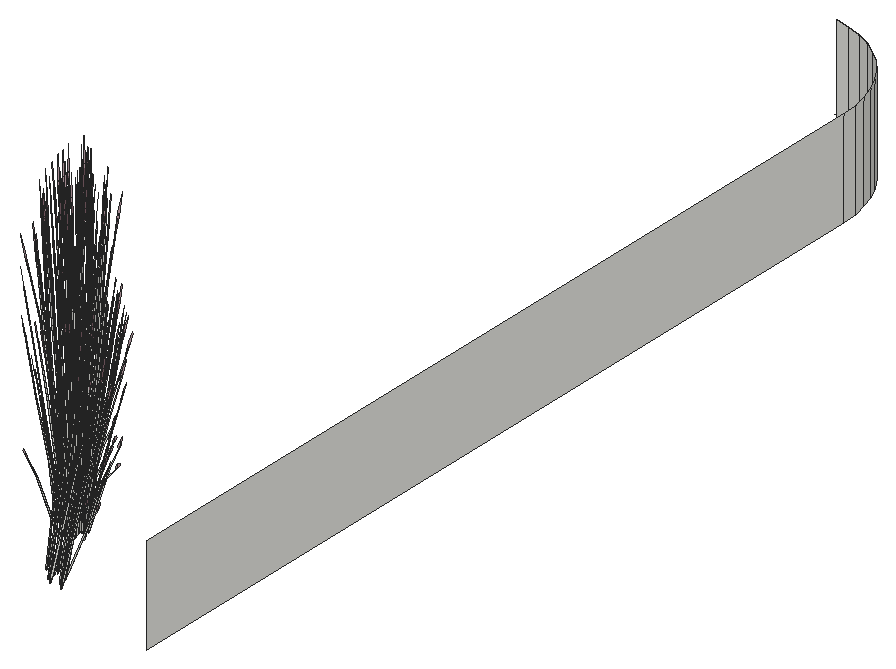
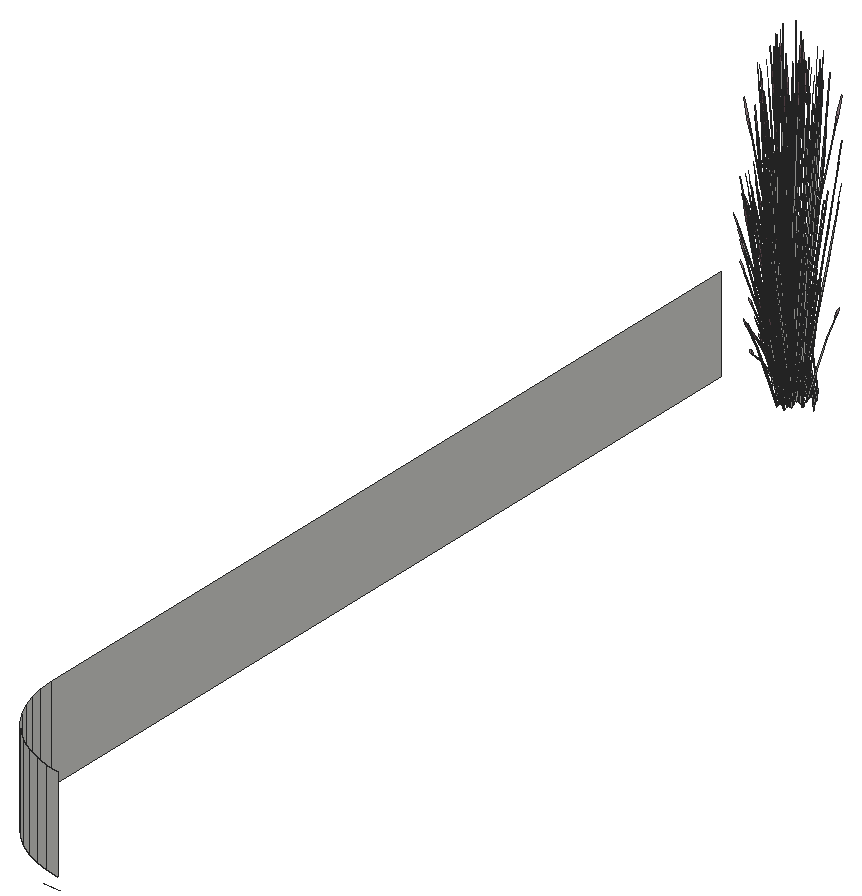
# SketchUp Ruby script. Lengths in inches.
U = 1.inch
M = Sketchup.active_model
def pt(a) = Geom::Point3d.new(a.map { |v| v * U })
def face(e, loops, mat)
  f = e.add_face(loops[0].map { |a| pt(a) })
  loops[1..].each { |l| e.add_face(l.map { |a| pt(a) }).erase! }
  f.material = f.back_material = mat if mat
  f
end
# faces: each face lists its corners as indices into pts; further lists are holes
def faces(e, pts, list, mat = nil) = list.each { |f| face(e, (f[0].is_a?(Array) ? f : [f]).map { |l| l.map { |i| pts[i] } }, mat) }
# xy, xz, yz: faces in a plane at the given z, y or x. An outline is a flat list of corners, or four numbers for a rectangle; further outlines are holes
def ring(l) = l.size == 4 ? [[l[0], l[1]], [l[2], l[1]], [l[2], l[3]], [l[0], l[3]]] : l.each_slice(2).to_a
def flat(e, list, mat, &to3) = list.each { |f| face(e, (f[0].is_a?(Array) ? f : [f]).map { |l| ring(l).map { |u, v| to3.(u, v) } }, mat) }
def xy(e, z, list, mat = nil) = flat(e, list, mat) { |x, y| [x, y, z] }
def xz(e, y, list, mat = nil) = flat(e, list, mat) { |x, z| [x, y, z] }
def yz(e, x, list, mat = nil) = flat(e, list, mat) { |y, z| [x, y, z] }
def lines(e, pts, list) = list.each { |a, b| e.add_line(pt(pts[a]), pt(pts[b])) }
# prism: a flat outline (further loops are holes) pulled along v
def prism(e, loops, v, mat = nil)
  f = face(e, loops, mat); d = Geom::Vector3d.new(v.map { |x| x * U })
  f.pushpull(f.normal.samedirection?(d) ? d.length : -d.length)
end
def box(e, o, s, mat = nil) = prism(e, [[o, [o[0] + s[0], o[1], o[2]], [o[0] + s[0], o[1] + s[1], o[2]], [o[0], o[1] + s[1], o[2]]]], [0, 0, s[2]], mat)
def at(x, y, z, deg = 0) = Geom::Transformation.translation(pt([x, y, z])) * Geom::Transformation.rotation(ORIGIN, Z_AXIS, deg.degrees)
def axes(o, x, y, z) = Geom::Transformation.new([*x, 0, *y, 0, *z, 0, *pt(o).to_a, 1])
def part(name) = M.definitions.add(name)
# library, detail: a bought-in or finely detailed component or shape, given as its bounding box
def library(name, o, s) = part(name).tap { |d| box(d.entities, o, s) }
def detail(e, o, s) = box(e.add_group.entities, o, s)
def put(e, d, t, mat = nil) = e.add_instance(d, t).tap { |i| i.material = mat if mat }
def group(e, t, mat = nil) = e.add_group.tap { |g| g.transformation = t; g.material = mat if mat }.entities
root = M.entities
M.materials.add("LightPink_Translucent").color = [144, 107, 117]
M.materials["LightPink_Translucent"].alpha = 0.75
c1 = part("blade")
p = [[2.15,0.21,22],[0,0.17,0],[0.09,0.45,0],[2.18,0.31,22],[2.29,0.31,22],[0.38,0.45,0],
  [2.48,0.24,33],[2.49,0.24,33],[2.48,0.22,33]]
faces(c1.entities,p,[[0,1,2,3],[4,5,2,3],[6,3,4,7],[8,0,3,6]])
c2 = part("seeds")
p = [[0.3,-0.1,1.38],[-0.01,-0.03,1.59],[-0.01,-0.03,0.03],[0.14,-0.07,-0.07],[0.29,-0.03,3],[0.15,0.01,3.11]]
faces(c2.entities,p,[[0,1,2,3],[1,0,4,5]],"LightPink_Translucent")
c3 = part("blade with seeds")
put(c3.entities,c1,at(0,0,0))
put(c3.entities,c2,axes([2.4,0.25,30.99],[1.5799,-0.05474,1.17369],[-0.12525,1.92788,0.29478],[-0.07173,-0.02425,1.56792]))
yz(root,375.57,[[661.9,618,822.84,636]])
p = [[375.39,825.68,618],[375.57,822.84,618],[375.57,822.84,636],[375.39,825.68,636],[374.85,828.375,618],[374.85,828.375,636],
  [373.97,830.97,618],[373.97,830.97,636],[372.76,833.4375,618],[372.76,833.4375,636],[371.23,835.72,618],[371.23,835.72,636],
  [369.42,837.79,618],[369.42,837.79,636],[367.36,839.6,618],[367.36,839.6,636],[365.07,841.12,618],[365.07,841.12,636],
  [362.61,842.34,618],[362.61,842.34,636],[360.01,843.22,618],[360.01,843.22,636],[357.59,843.7,618],[357.59,843.7,636],
  [357.71,846.74,618],[354.57,846.94,618],[357.88,846.7,618]]
faces(root,p,[[0,1,2,3],[4,0,3,5],[6,4,5,7],[8,6,7,9],[10,8,9,11],[12,10,11,13],[14,12,13,15],[16,14,15,17],
  [18,16,17,19],[20,18,19,21],[22,20,21,23]])
lines(root,p,[[24,25],[26,24]])
put(root,c3,axes([356.22,664.375,622.68],[0.34695,0.11691,-0.51099],[-0.11892,0.40083,-0.3958],[0.03181,0.16138,0.97773]))
put(root,c3,axes([357.33,664.56,620.82],[0.32063,-0.08258,0.06507],[0.07371,0.33271,-0.86304],[-0.02033,0.16842,0.7736]))
put(root,c3,axes([356.42,663.55,621.875],[-0.08068,-0.14973,1.71376],[0.3728,-0.12606,0.13857],[0.08426,0.23506,0.73262]))
put(root,c3,axes([358.35,664.39,622.68],[0.34695,0.11691,-0.51099],[-0.11892,0.40083,-0.3958],[0.03181,0.16138,0.97773]))
put(root,c3,axes([358.55,663.5625,621.875],[-0.08068,-0.14973,1.71376],[0.3728,-0.12606,0.13857],[0.08426,0.23506,0.73262]))
put(root,c3,axes([353.5,669.76,628.32],[0.16041,-0.29625,0.0643],[0.22843,0.17248,0.50621],[-0.07385,-0.09498,0.77189]))
put(root,c3,axes([352.875,669.72,625.08],[-0.03419,0.06144,1.76342],[-0.3455,0.13246,-0.26939],[-0.08346,-0.12049,0.30037]))
put(root,c3,axes([356.0625,664.62,622.53],[-0.1064,0.35863,-0.35414],[-0.31043,-0.1046,0.4572],[0.02846,0.14439,0.87481]))
put(root,c3,axes([358.19,664.63,622.53],[-0.1064,0.35863,-0.35414],[-0.31043,-0.1046,0.4572],[0.02846,0.14439,0.87481]))
put(root,c3,axes([353.44,671.41,625.6875],[-0.14494,-0.47823,-0.69835],[0.41752,-0.17223,-0.18329],[-0.01602,-0.16194,1.54149]))
put(root,c3,axes([355.38,669.95,625.08],[-0.05283,-0.03674,1.76342],[-0.13569,-0.41045,-0.26939],[0.09154,-0.11138,0.30037]))
put(root,c3,axes([355.39,663.93,623.34],[-0.00918,0.43138,-0.7886],[-0.38672,-0.02897,0.09517],[-0.04081,0.18275,1.11556]))
put(root,c3,axes([357.52,663.94,623.34],[-0.00918,0.43138,-0.7886],[-0.38672,-0.02897,0.09517],[-0.04081,0.18275,1.11556]))
put(root,c3,axes([354.38,665.06,622.71],[0.04004,-0.02816,1.77383],[0.33095,0.18728,-0.16761],[-0.00778,0.15594,0.31391]))
put(root,c3,axes([356.51,665.07,622.71],[0.04004,-0.02816,1.77383],[0.33095,0.18728,-0.16761],[-0.00778,0.15594,0.31391]))
put(root,c3,axes([354.29,670.04,628.64],[-0.1064,0.35863,0.35414],[-0.31043,-0.1046,-0.4572],[-0.02846,-0.14439,0.87481]))
put(root,c3,axes([353.32,670.1,628.27],[-0.34827,0.11086,-0.51099],[-0.06092,-0.41983,-0.3958],[-0.09354,-0.12031,0.97773]))
put(root,c3,axes([355.08,670.19,628.32],[0.25132,0.3182,0.48003],[-0.2669,0.27442,0.3958],[0.04636,-0.14929,0.9933]))
put(root,c3,axes([355.76,663.62,621.875],[-0.00864,-0.17899,1.71376],[0.37441,0.11874,0.13857],[-0.02316,0.25508,0.73262]))
put(root,c3,axes([357.89,663.64,621.875],[-0.00864,-0.17899,1.71376],[0.37441,0.11874,0.13857],[-0.02316,0.25508,0.73262]))
put(root,c3,axes([353.57,669.73,629.02],[-0.23555,0.44708,-0.13619],[-0.34112,-0.25757,-0.75594],[-0.11858,-0.12631,1.14864]))
put(root,c3,axes([355.18,670.22,628.32],[0.29004,0.02173,0.0643],[-0.00795,0.32812,0.50621],[0.03035,-0.12569,0.77189]))
put(root,c3,axes([354.96,670.44,628.64],[-0.23881,0.24554,0.35414],[-0.22606,-0.28036,-0.4572],[0.0344,-0.14245,0.87481]))
put(root,c3,axes([356.09,664.3,622.98],[0.16845,0.3792,-0.71045],[-0.34676,0.21133,0.08574],[0.03939,0.18322,1.00501]))
put(root,c3,axes([355.38,671.1,628.57],[0.18436,-0.36797,-0.71045],[0.32306,0.26151,0.08574],[0.11008,-0.13332,1.00501]))
put(root,c3,axes([358.22,664.3125,622.98],[0.16845,0.3792,-0.71045],[-0.34676,0.21133,0.08574],[0.03939,0.18322,1.00501]))
put(root,c3,axes([353.39,670.03,625.96],[-0.22066,-0.46731,0],[0.36918,-0.26061,-0.51607],[0.08408,-0.05936,1.63711]))
put(root,c3,axes([355.37,670.93,628.27],[-0.09067,-0.42583,-0.51099],[0.34336,-0.07449,-0.3958],[0.0984,-0.11438,0.97773]))
put(root,c3,axes([353.87,669.47,625.72],[-0.2439,0.26754,-0.03893],[-0.22348,-0.29302,-0.17649],[-0.01573,-0.08303,0.58215]))
put(root,c3,axes([355.12,664.89,620.59],[0.11138,-0.07357,1.43002],[0.27499,0.22183,-0.30754],[-0.08185,0.19194,0.61141]))
put(root,c3,axes([357.25,664.91,620.59],[0.11138,-0.07357,1.43002],[0.27499,0.22183,-0.30754],[-0.08185,0.19194,0.61141]))
put(root,c3,axes([355.84,665.25,622.72],[0.04474,0.0751,1.74944],[0.36104,0.0295,-0.27667],[0.03631,0.16562,0.14031]))
put(root,c3,axes([357.97,665.27,622.72],[0.04474,0.0751,1.74944],[0.36104,0.0295,-0.27667],[0.03631,0.16562,0.14031]))
put(root,c3,axes([355.53,671.24,628.62],[-0.32648,-0.25715,-0.1216],[0.18809,-0.3724,-0.67495],[0.09224,-0.12945,1.02557]))
put(root,c3,axes([354.19,672.64,626.91],[0.305,0.18805,1.51261],[-0.29879,0.40513,0.59816],[-0.13384,-0.24012,1.26806]))
put(root,c3,axes([353.54,670.1,628.64],[0.05451,0.37564,0.35414],[-0.31161,0.09919,-0.4572],[-0.0837,-0.10765,0.87481]))
put(root,c3,axes([352.59,671.34,625.61],[0,-0.46636,-0.49651],[0.39487,0,0],[0,-0.10622,1.57504]))
put(root,c3,axes([353.6875,669.96,625.61],[0.33032,-0.23318,-0.49651],[0.19744,0.41812,0],[0.07523,-0.05311,1.57504]))
put(root,c3,axes([355.65,670.77,626.18],[-0.12609,-0.01381,1.43002],[-0.12917,-0.37055,-0.30754],[0.1549,-0.10482,0.61141]))
put(root,c3,axes([356.34,671.125,628.3],[-0.0461,-0.00354,1.77383],[-0.19143,-0.37951,-0.16761],[0.07688,-0.12478,0.31391]))
put(root,c3,axes([355.26,664.53,621.36],[0.00775,-0.24075,1.54345],[0.34877,0.12716,0.21329],[-0.03022,0.25658,0.72882]))
put(root,c3,axes([357.39,664.55,621.36],[0.00775,-0.24075,1.54345],[0.34877,0.12716,0.21329],[-0.03022,0.25658,0.72882]))
put(root,c3,axes([354.08,670.92,625.65],[0.23773,-0.35053,-0.62353],[0.29532,0.31785,-0.16365],[0.09526,-0.08744,1.37633]))
put(root,c3,axes([355.79,670.08,626.35],[-0.11756,0.2374,1.1486],[-0.10105,-0.31895,0.84392],[0.09709,-0.07992,0.25299]))
put(root,c3,axes([355.625,670.98,628.12],[0.30722,-0.06665,-0.35414],[0.08112,0.381,0.4572],[0.08804,-0.10234,0.87481]))
put(root,c3,axes([353.67,671.53,625.8],[0.17124,-0.42022,-0.44739],[0.35581,0.20224,0.21531],[0,-0.09687,1.43643]))
put(root,c3,axes([353.82,671.32,626.25],[-0.04113,-0.53214,-0.29095],[0.42835,-0.03218,-0.50002],[0.07543,-0.07088,1.59708]))
put(root,c3,axes([352.76,671.35,625.62],[0.24637,-0.29097,-0.30978],[0.24637,0.29097,0.30978],[0,-0.09372,1.38974]))
put(root,c3,axes([352.66,669.96,625.72],[-0.10181,0.3808,-0.03893],[-0.31336,-0.11714,-0.17649],[-0.04758,-0.06228,0.58215]))
put(root,c3,axes([355.375,671.2,628.64],[-0.30722,0.06665,0.35414],[-0.08112,-0.381,-0.4572],[0.08804,-0.10234,0.87481]))
put(root,c3,axes([353.62,671.88,626.25],[-0.39748,-0.22252,-0.29095],[0.19139,-0.46966,-0.50002],[-0.01249,-0.11531,1.59708]))
put(root,c3,axes([352.49,671.69,625.96],[-0.44133,0,0],[0,-0.52122,-0.51607],[0,-0.11871,1.63711]))
put(root,c3,axes([353.76,670.14,625.62],[0.32928,0.11539,-0.30978],[-0.08291,0.40636,0.30978],[0.06638,-0.04686,1.38974]))
put(root,c3,axes([355.65,671.14,628.32],[0.2423,0.19613,0.0643],[-0.14107,0.2793,0.50621],[0.07768,-0.0903,0.77189]))
put(root,c3,axes([355.59,671.06,628.32],[0.08753,0.42921,0.48003],[-0.34336,0.07449,0.3958],[0.1012,-0.10094,0.9933]))
put(root,c3,axes([356.51,671.58,628.3],[0.04898,-0.07104,1.74944],[-0.06269,-0.43574,-0.27667],[0.12289,-0.08262,0.14031]))
put(root,c3,axes([352.83,671.56,625.92],[-0.32829,0.39208,0.30756],[-0.32849,-0.38796,-0.36492],[-0.01146,-0.11134,1.64885]))
put(root,c3,axes([353.88,671.74,626.02],[0.39767,0.22603,0.24065],[-0.19139,0.46966,0.50002],[0,-0.10827,1.60543]))
put(root,c3,axes([353.72,672.375,626.03],[0.09355,-0.55261,-0.23429],[0.44354,0.09633,0.51271],[-0.0775,-0.07631,1.5644]))
put(root,c3,axes([352.92,670.61,628.64],[0.20082,0.29199,0.35414],[-0.2293,0.2764,-0.4572],[-0.1165,-0.04206,0.87481]))
put(root,c3,axes([353.75,671.42,626.31],[-0.38326,0.02879,0.44739],[-0.03466,-0.47788,-0.21531],[0.06861,-0.04843,1.43643]))
put(root,c3,axes([352.76,671.77,626.07],[0,0.46636,0.49651],[-0.39487,0,0],[0,-0.10622,1.57504]))
put(root,c3,axes([355.55,672.24,628.62],[-0.17758,-0.42229,-0.1216],[0.31518,-0.20752,-0.67495],[0.13282,-0.05572,1.02557]))
put(root,c3,axes([355.53,671.875,628.27],[0.09562,-0.42421,-0.51099],[0.32782,0.1454,-0.3958],[0.13199,-0.0389,0.97773]))
put(root,c3,axes([355.01,670.15,625.97],[0.22066,-0.46731,0],[0.36918,0.26061,-0.51607],[0.08408,0.05936,1.63711]))
put(root,c3,axes([353.69,672.15,625.8],[-0.21202,-0.39143,-0.44739],[0.32115,-0.27564,0.21531],[-0.06861,-0.04843,1.43643]))
put(root,c3,axes([353.74,671.6,625.95],[0.15345,0.52148,0.45755],[-0.43845,0.18134,0.17955],[0.00536,-0.09582,1.58856]))
put(root,c3,axes([355.88,672,625.57],[-0.22732,0.05597,1.41583],[-0.03618,-0.44548,0.08104],[0.15921,-0.06743,0.80566]))
put(root,c3,axes([356.3,671.6,625.85],[-0.21881,-0.29821,-0.06488],[0.23965,-0.27324,-0.29416],[0.0679,-0.01924,0.97024]))
put(root,c3,axes([353.66,672.01,626.31],[-0.17124,0.42022,0.44739],[-0.35581,-0.20224,-0.21531],[0,-0.09687,1.43643]))
put(root,c3,axes([354.29,671.64,625.79],[0,-0.53961,0],[0.44133,0,0],[0,0,1.79456]))
put(root,c3,axes([354.82,670.39,626.07],[-0.33032,-0.23318,0.49651],[0.19744,-0.41812,0],[0.07523,0.05311,1.57504]))
put(root,c3,axes([355.47,672.03,628.57],[0.31014,-0.20596,-0.71045],[0.17284,0.42397,0.08574],[0.14985,-0.04816,1.00501]))
put(root,c3,axes([353.5,672.3,625.65],[-0.36714,-0.07646,-0.62353],[0.07747,-0.47163,-0.16365],[-0.10956,-0.05715,1.37633]))
put(root,c3,axes([354.08,671.3,625.95],[-0.29264,0.42323,0.45755],[-0.34767,-0.3736,0.17955],[0.07055,-0.04224,1.58856]))
put(root,c3,axes([354.4,672.06,625.89],[-0.32829,-0.4014,-0.06131],[0.32849,-0.40164,0],[-0.01146,-0.01402,1.75571]))
put(root,c3,axes([353.57,670.6,626.0625],[-0.10196,0.46348,0.17642],[-0.3731,-0.13116,0.35086],[0.06445,-0.00226,1.60407]))
put(root,c3,axes([355.42,672.11,628.64],[-0.29332,-0.1301,0.35414],[0.08555,-0.37955,-0.4572],[0.11809,-0.0348,0.87481]))
put(root,c3,axes([353.42,670.98,625.18],[-0.3474,0.18671,1.28929],[-0.11057,-0.53572,0.50096],[0.21332,0.00891,1.46642]))
put(root,c3,axes([354.35,671.12,626.2],[0.06809,-0.4162,0.1448],[0.33266,0.07225,-0.41347],[0.06054,0.04274,1.26744]))
put(root,c3,axes([353.77,672.11,625.95],[0.44609,0.09826,0.45755],[-0.09078,0.55493,0.17955],[-0.06519,-0.05359,1.58856]))
put(root,c3,axes([356.13,671.71,625.08],[-0.01845,-0.0708,1.76342],[0.12793,-0.41416,-0.26939],[0.12905,-0.00596,0.30037]))
put(root,c3,axes([354.21,671.23,626.31],[-0.21202,-0.39143,0.44739],[0.32115,-0.27564,-0.21531],[0.06861,0.04843,1.43643]))
put(root,c3,axes([353.11,673.02,625.62],[-0.08291,-0.40636,-0.30978],[0.32928,-0.11539,0.30978],[-0.06638,-0.04686,1.38974]))
put(root,c3,axes([353.53,672.99,626.0625],[0.37926,-0.12378,0.17642],[0.09365,0.46065,0.35086],[-0.03382,-0.06712,1.60407]))
put(root,c3,axes([354.32,671.25,626.25],[0.35635,-0.30962,-0.29095],[0.23697,0.43749,-0.50002],[0.08792,0.04443,1.59708]))
put(root,c3,axes([355.73,672.07,628.12],[0.29332,0.1301,-0.35414],[-0.08555,0.37955,0.4572],[0.11809,-0.0348,0.87481]))
put(root,c3,axes([353.02,673.19,625.61],[-0.33032,-0.23318,-0.49651],[0.19744,-0.41812,0],[-0.07523,-0.05311,1.57504]))
put(root,c3,axes([355.21,670.43,625.61],[0.33032,0.23318,-0.49651],[-0.19744,0.41812,0],[0.07523,0.05311,1.57504]))
put(root,c3,axes([354.59,671.76,625.79],[0.39487,0,0],[0,0.48281,0],[0,0,1.78407]))
put(root,c3,axes([353.92,672.37,626.25],[-0.35635,0.30962,-0.29095],[-0.23697,-0.43749,-0.50002],[-0.08792,-0.04443,1.59708]))
put(root,c3,axes([354.7,670.63,626.0625],[-0.37926,0.12378,0.17642],[-0.09365,-0.46065,0.35086],[0.03382,0.06712,1.60407]))
put(root,c3,axes([354.93,671.6,627.46],[-0.14639,0.01056,1.71376],[0.09712,-0.45778,0.13857],[0.20862,0.02831,0.73262]))
put(root,c3,axes([355.12,670.61,625.62],[0.08291,0.40636,-0.30978],[-0.32928,0.11539,0.30978],[0.06638,0.04686,1.38974]))
put(root,c3,axes([355.6875,672.23,628.32],[0.12963,0.31798,0.0643],[-0.23638,0.15564,0.50621],[0.1042,-0.03071,0.77189]))
put(root,c3,axes([354.46,671.52,625.97],[-0.44609,-0.09826,0.49198],[0.09078,-0.55493,0.19306],[0.06519,0.05359,1.70813]))
put(root,c3,axes([355.66,672.12,628.32],[-0.09971,0.42522,0.48003],[-0.32782,-0.1454,0.3958],[0.12892,-0.02555,0.9933]))
put(root,c3,axes([354.1,672.89,625.79],[-0.11516,-0.40207,0],[0.32884,-0.1408,0],[0,0,1.54371]))
put(root,c3,axes([353.88,672.5,626.2],[-0.06809,0.4162,0.1448],[-0.33266,-0.07225,-0.41347],[-0.06054,-0.04274,1.26744]))
put(root,c3,axes([354.53,672.83,625.77],[0.37054,-0.15823,-0.19198],[0.1302,0.45581,0.00008],[0.0409,-0.01749,1.73897]))
put(root,c3,axes([354.66,673.02,626.0625],[0.10196,-0.46348,0.17642],[0.3731,0.13116,0.35086],[-0.06445,0.00226,1.60407]))
put(root,c3,axes([354.58,671.97,625.8],[0.24637,0.30123,0],[-0.24637,0.30123,0],[0,0,1.69266]))
put(root,c3,axes([355.25,671.84,626.0625],[-0.2773,-0.3397,0.17642],[0.27945,-0.32949,0.35086],[-0.03063,0.06937,1.60407]))
put(root,c3,axes([354.73,671.32,625.65],[0.36714,0.07646,-0.62353],[-0.07747,0.47163,-0.16365],[0.10956,0.05715,1.37633]))
put(root,c3,axes([356.35,672.15,626.35],[-0.21807,0.07699,1.1486],[0.10265,-0.31819,0.84392],[0.11568,0.02177,0.25299]))
put(root,c3,axes([354.02,673.07,625.78],[-0.35581,-0.20937,0],[0.17124,-0.43505,0],[0,0,1.62707]))
put(root,c3,axes([354.32,672.51,626.05],[-0.34464,-0.37536,-0.25192],[0.29,-0.42149,0.5513],[-0.0928,0.04391,1.68216]))
put(root,c3,axes([353.41,673.23,626.07],[0.33032,0.23318,0.49651],[-0.19744,0.41812,0],[-0.07523,-0.05311,1.57504]))
put(root,c3,axes([354.58,671.62,626.31],[0.17124,-0.42022,0.44739],[0.35581,0.20224,-0.21531],[0,0.09687,1.43643]))
put(root,c3,axes([356.25,673.49,628.3],[-0.03191,-0.04083,1.77383],[0.06981,-0.43764,-0.16761],[0.12571,-0.02796,0.31391]))
put(root,c3,axes([354.51,671.86,625.88],[0,0.53934,-0.05637],[-0.44133,0,0],[0,0.01695,1.79368]))
put(root,c3,axes([354.54,671.47,625.8],[0.21202,0.39143,-0.44739],[-0.32115,0.27564,0.21531],[0.06861,0.04843,1.43643]))
put(root,c3,axes([355.98,673.13,627.52],[-0.06755,-0.39203,-0.03492],[0.31928,-0.09013,-0.15832],[0.06667,0.02485,0.52218]))
put(root,c3,axes([353.22,673.47,625.96],[-0.22066,0.46731,0],[-0.36918,-0.26061,-0.51607],[-0.08408,-0.05936,1.63711]))
put(root,c3,axes([355.15,673.12,628.62],[0.0189,-0.47427,-0.1216],[0.35781,0.01296,-0.67495],[0.13781,0.03295,1.02557]))
put(root,c3,axes([355.47,671.85,626.07],[0,-0.46636,0.49651],[0.39487,0,0],[0,0.10622,1.57504]))
put(root,c3,axes([354.48,672.2,626.31],[0.38326,-0.02879,0.44739],[0.03466,0.47788,-0.21531],[-0.06861,0.04843,1.43643]))
put(root,c3,axes([354.72,671.71,626.2],[0.32884,-0.136,0.1448],[0.11516,0.38837,-0.41347],[0,0.08547,1.26744]))
put(root,c3,axes([355.09,672.93,628.64],[-0.20082,-0.29199,0.35414],[0.2293,-0.2764,-0.4572],[0.1165,0.04206,0.87481]))
put(root,c3,axes([354.14,672.43,625.8],[-0.38326,0.02879,-0.44739],[-0.03466,-0.47788,0.21531],[-0.06861,0.04843,1.43643]))
put(root,c3,axes([355.95,672.66,626.18],[-0.085,-0.1147,1.43002],[0.1106,-0.37943,-0.30754],[0.17198,0.0514,0.61141]))
put(root,c3,axes([354.43,673.08,625.79],[0.35581,0.20937,0],[-0.17124,0.43505,0],[0,0,1.74954]))
put(root,c3,axes([355.46,672.83,628.3],[0.07571,-0.00789,1.74944],[0.20767,-0.36231,-0.27667],[0.13467,0.04783,0.14031]))
put(root,c3,axes([354.57,673.54,625.78],[-0.21791,-0.46895,-0.05142],[0.36918,-0.26061,0.51607],[-0.09097,0.04465,1.6363]))
put(root,c3,axes([354.49,672.4,626.2],[0.26075,0.2802,0.1448],[-0.2175,0.31612,-0.41347],[-0.06054,0.04274,1.26744]))
put(root,c3,axes([355.17,672.89,628.57],[0.35281,0.01123,-0.71045],[-0.0237,0.47284,0.08574],[0.14947,0.0499,1.00501]))
put(root,c3,axes([354.77,673.27,626.07],[0.33032,-0.23318,0.49651],[0.19744,0.41812,0],[-0.07523,0.05311,1.57504]))
put(root,c3,axes([354.3,672.9,625.88],[0.15345,0.53576,-0.06012],[-0.43845,0.18773,0],[0.00536,0.01871,1.72173]))
put(root,c3,axes([354.47,673.48,625.62],[-0.32928,-0.11539,-0.30978],[0.08291,-0.40636,0.30978],[-0.06638,0.04686,1.38974]))
put(root,c3,axes([352.64,672.34,628.64],[0.30722,-0.06665,0.35414],[0.08112,0.381,-0.4572],[-0.08804,0.10234,0.87481]))
put(root,c3,axes([355.74,671.93,625.97],[0.44133,0,0],[0,0.52122,-0.51607],[0,0.11871,1.63711]))
put(root,c3,axes([355.57,672.2,625.79],[-0.44111,-0.00373,-0.04976],[0,-0.52122,0.49943],[-0.01386,0.11865,1.58352]))
put(root,c3,axes([354.61,671.74,626.25],[0.39748,0.22252,-0.29095],[-0.19139,0.46966,-0.50002],[0.01249,0.11531,1.59708]))
put(root,c3,axes([355.38,673.08,628.12],[0.20082,0.29199,-0.35414],[-0.2293,0.2764,0.4572],[0.1165,0.04206,0.87481]))
put(root,c3,axes([355.47,672.27,625.62],[-0.24637,0.29097,-0.30978],[-0.24637,-0.29097,0.30978],[0,0.09372,1.38974]))
put(root,c3,axes([354.41,672.3,626.25],[0.04113,0.53214,-0.29095],[-0.42835,0.03218,-0.50002],[-0.07543,0.07088,1.59708]))
put(root,c3,axes([355.28,673.2,628.32],[-0.01777,0.35463,0.0643],[-0.26836,-0.00972,0.50621],[0.1028,0.03711,0.77189]))
put(root,c3,axes([354.57,672.09,625.8],[-0.17124,0.42022,-0.44739],[-0.35581,-0.20224,0.21531],[0,0.09687,1.43643]))
put(root,c3,axes([355.3,673.08,628.32],[-0.26024,0.30729,0.48003],[-0.22444,-0.32634,0.3958],[0.1221,0.05668,0.9933]))
put(root,c3,axes([351.95,673.42,629.23],[0.31145,0.12449,-0.06488],[-0.0958,0.38314,-0.29416],[-0.05094,0.05817,0.97024]))
put(root,c3,axes([354.15,672.71,625.65],[-0.23773,0.35053,-0.62353],[-0.29532,-0.31785,-0.16365],[-0.09526,0.08744,1.37633]))
put(root,c3,axes([354.47,673.4375,628.64],[-0.05451,-0.37564,0.35414],[0.31161,-0.09919,-0.4572],[0.0837,0.10765,0.87481]))
put(root,c3,axes([354.58,673.3,625.92],[0.44186,0.15158,0.30756],[-0.11054,0.54181,-0.36492],[-0.07313,0.06781,1.64885]))
put(root,c3,axes([354.55,673.66,625.61],[-0.33032,0.23318,-0.49651],[-0.19744,-0.41812,0],[-0.07523,0.05311,1.57504]))
put(root,c3,axes([355.64,672.28,625.61],[0,0.46636,-0.49651],[-0.39487,0,0],[0,0.10622,1.57504]))
put(root,c3,axes([354.66,672.34,627.46],[-0.1311,-0.08035,1.71376],[0.27131,-0.33708,0.13857],[0.16909,0.15206,0.73262]))
put(root,c3,axes([354.68,671.28,628.0625],[-0.30498,-0.24231,1.38283],[0.32203,-0.37727,0.59665],[0.0984,0.22736,1.33663]))
put(root,c3,axes([352.48,672.3,628.62],[0.32648,0.25715,-0.1216],[-0.18809,0.3724,-0.67495],[-0.09224,0.12945,1.02557]))
put(root,c3,axes([355.14,673.25,626.35],[-0.19872,-0.13409,1.1486],[0.2566,-0.13625,0.84392],[0.06921,0.11541,0.25299]))
put(root,c3,axes([354.44,673.63,628.62],[0.21031,-0.39918,-0.1216],[0.30457,0.22997,-0.67495],[0.10587,0.11278,1.02557]))
put(root,c3,axes([353.06,673.09,628.64],[0.23881,-0.24554,0.35414],[0.22606,0.28036,-0.4572],[-0.0344,0.14245,0.87481]))
put(root,c3,axes([354.85,673.59,625.96],[0.22066,0.46731,0],[-0.36918,0.26061,-0.51607],[-0.08408,0.05936,1.63711]))
put(root,c3,axes([354.17,673.96,628.3],[0.00104,-0.05646,1.77383],[0.30246,-0.2491,-0.16761],[0.10506,0.08891,0.31391]))
put(root,c3,axes([355.2,673.75,625.08],[0.02571,-0.06733,1.76342],[0.32373,-0.19829,-0.26939],[0.09815,0.10263,0.30037]))
put(root,c3,axes([354.66,671.74,626.43],[-0.00964,-0.43909,1.41272],[0.43635,0.11382,0.59816],[-0.1032,0.24027,1.3335]))
put(root,c3,axes([354.77,672.22,625.68],[0.12941,0.42699,-0.69212],[-0.37279,0.15378,-0.18165],[0.0143,0.14459,1.52773]))
put(root,c3,axes([352.84,673.32,628.32],[-0.29004,-0.02173,0.0643],[0.00795,-0.32812,0.50621],[-0.03035,0.12569,0.77189]))
put(root,c3,axes([352.93,673.35,628.32],[-0.25132,-0.3182,0.48003],[0.2669,-0.27442,0.3958],[-0.04636,0.14929,0.9933]))
put(root,c3,axes([354.69,673.44,628.27],[0.34827,-0.11086,-0.51099],[0.06092,0.41983,-0.3958],[0.09354,0.12031,0.97773]))
put(root,c3,axes([353.73,673.5,628.64],[0.1064,-0.35863,0.35414],[0.31043,0.1046,-0.4572],[0.02846,0.14439,0.87481]))
put(root,c3,axes([355.17,673.86,626.26],[-0.22633,-0.01463,1.0506],[0.14947,-0.31064,0.58006],[0.08941,0.11036,0.8241]))
put(root,c3,axes([354.52,673.78,628.32],[-0.16041,0.29625,0.0643],[-0.22843,-0.17248,0.50621],[0.07385,0.09498,0.77189]))
put(root,c3,axes([354.14,674.78,629.23],[0.2439,-0.26754,-0.06488],[0.22348,0.29302,-0.29416],[0.01573,0.08303,0.97024]))
put(root,c3,axes([354.59,673.7,628.32],[-0.35104,0.10702,0.48003],[-0.06092,-0.41983,0.3958],[0.08256,0.12373,0.9933]))
put(root,c3,axes([354.43,673.11,626.18],[0.00623,-0.15459,1.43002],[0.29764,-0.17268,-0.30754],[0.09188,0.18503,0.61141]))
put(root,c3,axes([353.63,673.82,628.32],[-0.26007,0.1585,0.0643],[-0.12729,-0.28902,0.50621],[0.02512,0.1274,0.77189]))
put(root,c3,axes([352.93,673.44,628.12],[-0.23881,0.24554,-0.35414],[-0.22606,-0.28036,0.4572],[-0.0344,0.14245,0.87481]))
put(root,c3,axes([352.91,673.16,628.99],[0.3879,0.02311,-0.13498],[-0.0106,0.43749,-0.74919],[-0.02694,0.1685,1.13838]))
put(root,c3,axes([353.62,673.65,628.62],[0.34538,-0.21713,-0.1216],[0.16972,0.38536,-0.67495],[0.04557,0.16239,1.02557]))
put(root,c3,axes([353.72,673.79,628.65],[-0.34777,-0.12192,0.53283],[0.11892,-0.40083,0.43934],[0.0209,0.15763,1.10256]))
put(root,c3,axes([353.08,674.4,626.35],[-0.00913,-0.2773,1.1486],[0.22824,0.19778,0.84392],[-0.04489,0.13217,0.25299]))
put(root,c3,axes([353.69,673.73,625.08],[0.05712,-0.02538,1.76342],[0.34359,0.13968,-0.26939],[0.01005,0.15742,0.30037]))
put(root,c3,axes([353.17,673.33,628.59],[0.25266,0.31335,-0.5672],[-0.2669,0.27442,-0.43934],[-0.03844,0.15921,1.08528]))
put(root,c3,axes([352.9,673.8,626.41],[0.32063,-0.08258,0.06507],[0.07371,0.33271,-0.86304],[-0.02033,0.16842,0.7736]))
put(root,c3,axes([353.92,673.63,628.27],[0.34695,0.11691,-0.51099],[-0.11892,0.40083,-0.3958],[0.03181,0.16138,0.97773]))
put(root,c3,axes([354.12,672.8,627.46],[-0.08068,-0.14973,1.71376],[0.3728,-0.12606,0.13857],[0.08426,0.23506,0.73262]))
put(root,c3,axes([353.76,673.875,628.12],[-0.1064,0.35863,-0.35414],[-0.31043,-0.1046,0.4572],[0.02846,0.14439,0.87481]))
put(root,c3,axes([353.09,673.18,628.93],[-0.00918,0.43138,-0.7886],[-0.38672,-0.02897,0.09517],[-0.04081,0.18275,1.11556]))
put(root,c3,axes([352.08,674.32,628.3],[0.04004,-0.02816,1.77383],[0.33095,0.18728,-0.16761],[-0.00778,0.15594,0.31391]))
put(root,c3,axes([353.46,672.88,627.46],[-0.00864,-0.17899,1.71376],[0.37441,0.11874,0.13857],[-0.02316,0.25508,0.73262]))
put(root,c3,axes([353.79,673.55,628.57],[0.16845,0.3792,-0.71045],[-0.34676,0.21133,0.08574],[0.03939,0.18322,1.00501]))
put(root,c3,axes([352.82,674.15,626.18],[0.11138,-0.07357,1.43002],[0.27499,0.22183,-0.30754],[-0.08185,0.19194,0.61141]))
put(root,c3,axes([353.54,674.51,628.3],[0.04474,0.0751,1.74944],[0.36104,0.0295,-0.27667],[0.03631,0.16562,0.14031]))
put(root,c3,axes([352.96,673.79,626.95],[0.00775,-0.24075,1.54345],[0.34877,0.12716,0.21329],[-0.03022,0.25658,0.72882]))
